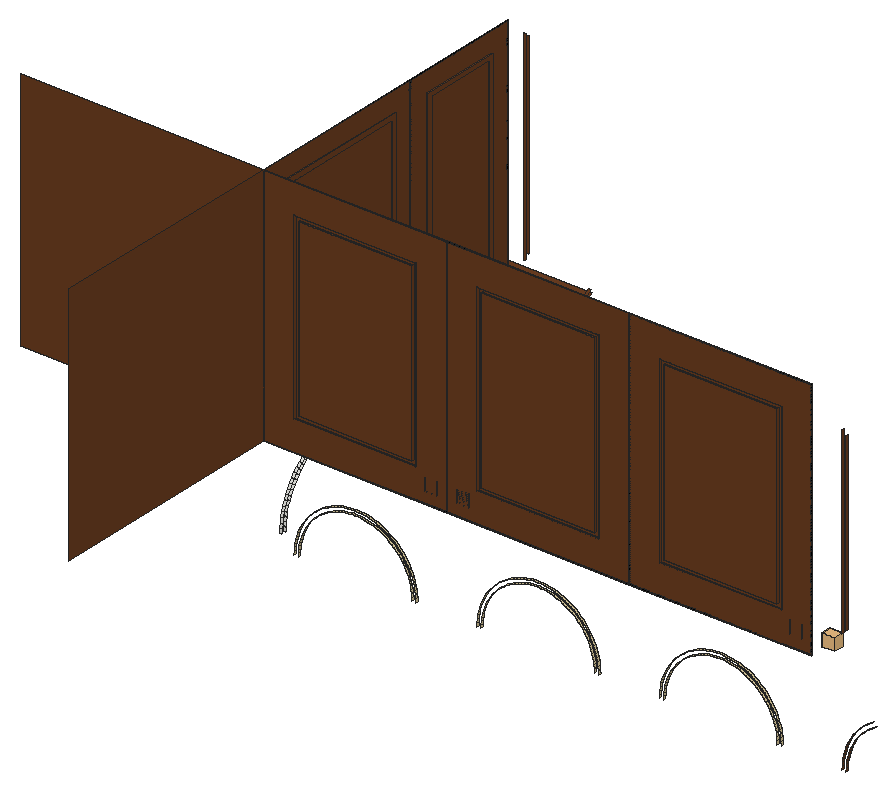
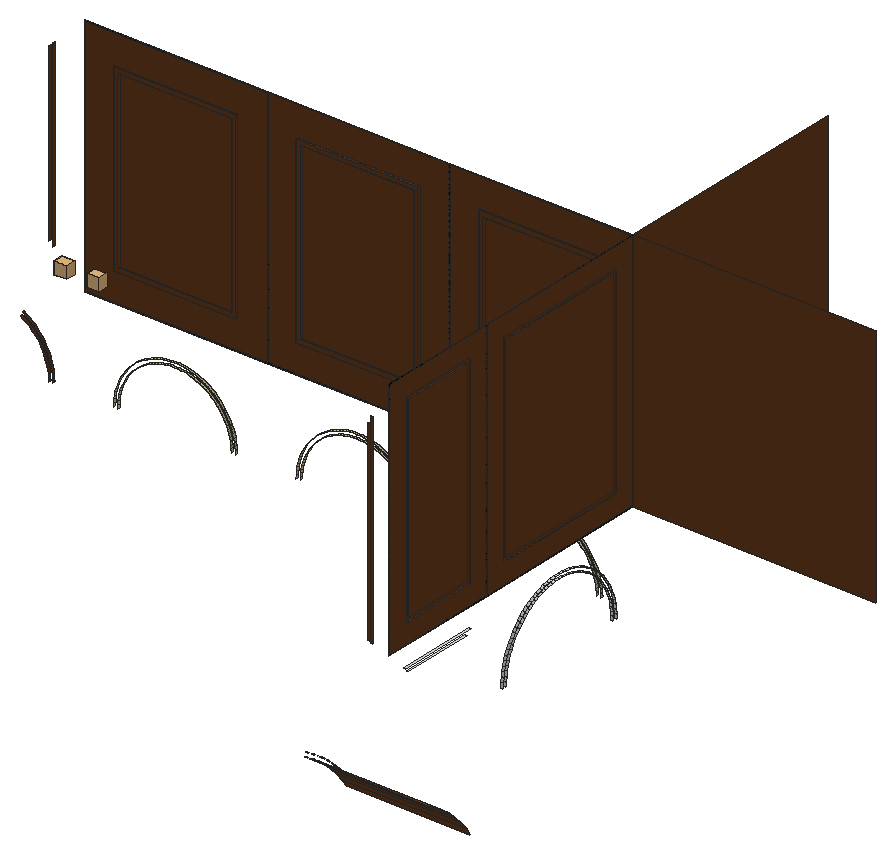
# SketchUp Ruby script. Lengths in inches.
U = 1.inch
M = Sketchup.active_model
def pt(a) = Geom::Point3d.new(a.map { |v| v * U })
def face(e, loops, mat)
  f = e.add_face(loops[0].map { |a| pt(a) })
  loops[1..].each { |l| e.add_face(l.map { |a| pt(a) }).erase! }
  f.material = f.back_material = mat if mat
  f
end
# faces: each face lists its corners as indices into pts; further lists are holes
def faces(e, pts, list, mat = nil) = list.each { |f| face(e, (f[0].is_a?(Array) ? f : [f]).map { |l| l.map { |i| pts[i] } }, mat) }
# xy, xz, yz: faces in a plane at the given z, y or x. An outline is a flat list of corners, or four numbers for a rectangle; further outlines are holes
def ring(l) = l.size == 4 ? [[l[0], l[1]], [l[2], l[1]], [l[2], l[3]], [l[0], l[3]]] : l.each_slice(2).to_a
def flat(e, list, mat, &to3) = list.each { |f| face(e, (f[0].is_a?(Array) ? f : [f]).map { |l| ring(l).map { |u, v| to3.(u, v) } }, mat) }
def xy(e, z, list, mat = nil) = flat(e, list, mat) { |x, y| [x, y, z] }
def xz(e, y, list, mat = nil) = flat(e, list, mat) { |x, z| [x, y, z] }
def yz(e, x, list, mat = nil) = flat(e, list, mat) { |y, z| [x, y, z] }
def lines(e, pts, list) = list.each { |a, b| e.add_line(pt(pts[a]), pt(pts[b])) }
# prism: a flat outline (further loops are holes) pulled along v
def prism(e, loops, v, mat = nil)
  f = face(e, loops, mat); d = Geom::Vector3d.new(v.map { |x| x * U })
  f.pushpull(f.normal.samedirection?(d) ? d.length : -d.length)
end
def box(e, o, s, mat = nil) = prism(e, [[o, [o[0] + s[0], o[1], o[2]], [o[0] + s[0], o[1] + s[1], o[2]], [o[0], o[1] + s[1], o[2]]]], [0, 0, s[2]], mat)
def at(x, y, z, deg = 0) = Geom::Transformation.translation(pt([x, y, z])) * Geom::Transformation.rotation(ORIGIN, Z_AXIS, deg.degrees)
def axes(o, x, y, z) = Geom::Transformation.new([*x, 0, *y, 0, *z, 0, *pt(o).to_a, 1])
def part(name) = M.definitions.add(name)
# library, detail: a bought-in or finely detailed component or shape, given as its bounding box
def library(name, o, s) = part(name).tap { |d| box(d.entities, o, s) }
def detail(e, o, s) = box(e.add_group.entities, o, s)
def put(e, d, t, mat = nil) = e.add_instance(d, t).tap { |i| i.material = mat if mat }
def group(e, t, mat = nil) = e.add_group.tap { |g| g.transformation = t; g.material = mat if mat }.entities
root = M.entities
M.materials.add("138_plaster painted wall texture-seamless").color = [214, 198, 153]
M.materials.add("[0137_Black]").color = [0, 0, 0]
M.materials.add("[Wood Veneer 01]").color = [104, 60, 32]
c1 = library("Group\#17",[0,0,0],[1.625,1.625,1.31])
xy(root,85.6,[[24,44.4,24.2,51.6]])
xy(root,86,[[24,44,24.2,52]])
xy(root,90,[[24,26,24.2,40],[24,44,24.2,52]],"[Wood Veneer 01]")
xy(root,90.4,[[24,26.4,24.2,39.6],[24,44.4,24.2,51.6]],"[Wood Veneer 01]")
xy(root,91,[[27,24,39,24.2],[45,24,57,24.2],[63,24,75,24.2]],"[Wood Veneer 01]")
xy(root,91.4,[[27.4,24,38.6,24.2],[45.4,24,56.6,24.2],[63.4,24,74.6,24.2]],"[Wood Veneer 01]")
xy(root,108.6,[[63.4,24,74.6,24.2]],"138_plaster painted wall texture-seamless")
xy(root,108.6,[[27.4,24,38.6,24.2],[45.4,24,56.6,24.2]],"[Wood Veneer 01]")
xy(root,109,[[27,24,39,24.2],[45,24,57,24.2],[63,24,75,24.2]],"[Wood Veneer 01]")
xy(root,109.6,[[24,26.4,24.2,39.6],[24,44.4,24.2,51.6]],"[Wood Veneer 01]")
xy(root,110,[[24,26,24.2,40],[24,44,24.2,52]],"[Wood Veneer 01]")
xz(root,24,[[[24,88,42,112],[24.1,88.1,41.9,111.9]],[[42,88,60,112],[42.1,88.1,59.9,111.9]],[[60,88,78,112],[60.1,88.1,77.9,111.9]]],"[0137_Black]")
xz(root,24,[[0,88,24,112],[[24.1,88.1,41.9,111.9],[27,91,39,109]],[[42.1,88.1,59.9,111.9],[45,91,57,109]],[[60.1,88.1,77.9,111.9],[63,91,75,109]],[27.4,91.4,38.6,108.6],
  [45.4,91.4,56.6,108.6],[63.4,91.4,74.6,108.6]],"[Wood Veneer 01]")
xz(root,24.2,[[[27,91,39,109],[27.4,91.4,38.6,108.6]],[[45,91,57,109],[45.4,91.4,56.6,108.6]],[[63,91,75,109],[63.4,91.4,74.6,108.6]]],"[Wood Veneer 01]")
xz(root,26,[[24,90,24.2,110]],"[Wood Veneer 01]")
xz(root,26.4,[[24,90.4,24.2,109.6]],"[Wood Veneer 01]")
xz(root,39.6,[[24,90.4,24.2,109.6]],"[Wood Veneer 01]")
xz(root,40,[[24,90,24.2,110]],"[Wood Veneer 01]")
xz(root,44,[[24,90,24.2,110]],"[Wood Veneer 01]")
xz(root,44.4,[[24,90.4,24.2,109.6]],"[Wood Veneer 01]")
xz(root,51.6,[[24,90.4,24.2,109.6]],"[Wood Veneer 01]")
xz(root,52,[[24,90,24.2,110]],"[Wood Veneer 01]")
xz(root,56,[[24,90,24.2,110]],"[Wood Veneer 01]")
xz(root,56.4,[[24,90.4,24.2,109.6]],"[Wood Veneer 01]")
yz(root,24,[[[24,88,42,112],[24.1,88.1,41.9,111.9]],[[42,88,54,112],[42.1,88.1,53.9,111.9]]],"[0137_Black]")
yz(root,24,[[0,88,24,112],[[24.1,88.1,41.9,111.9],[26,90,40,110]],[[42.1,88.1,53.9,111.9],[44,90,52,110]],[26.4,90.4,39.6,109.6],[44.4,90.4,51.6,109.6]],"[Wood Veneer 01]")
yz(root,24.2,[[[26,90,40,110],[26.4,90.4,39.6,109.6]],[[44,90,52,110],[44.4,90.4,51.6,109.6]]],"[Wood Veneer 01]")
yz(root,27,[[24,91,24.2,109]],"[Wood Veneer 01]")
yz(root,27.4,[[24,91.4,24.2,108.6]],"[Wood Veneer 01]")
yz(root,38.6,[[24,91.4,24.2,108.6]],"[Wood Veneer 01]")
yz(root,39,[[24,91,24.2,109]],"[Wood Veneer 01]")
yz(root,45,[[24,91,24.2,109]],"[Wood Veneer 01]")
yz(root,45.4,[[24,91.4,24.2,108.6]],"[Wood Veneer 01]")
yz(root,56.6,[[24,91.4,24.2,108.6]],"[Wood Veneer 01]")
yz(root,57,[[24,91,24.2,109]],"[Wood Veneer 01]")
yz(root,63,[[24,91,24.2,109]],"[Wood Veneer 01]")
yz(root,63.4,[[24,91.4,24.2,108.6]],"[Wood Veneer 01]")
yz(root,74.6,[[24,91.4,24.2,108.6]],"[Wood Veneer 01]")
yz(root,75,[[24,91,24.2,109]],"[Wood Veneer 01]")
yz(root,81,[[24,91,24.2,109]],"[Wood Veneer 01]")
yz(root,81.4,[[24,91.4,24.2,108.6]],"[Wood Veneer 01]")
p = [[12,59.625,79.5],[24.2,59.625,79.5],[24.2,59.03,78.67],[12,59.03,78.67],[24,59.31,79.74],[24,58.7,78.89],
  [24.2,58.7,78.89],[24.2,59.31,79.74],[27,24,79],[27.01,24,79.35],[27.01,24.2,79.35],[27,24.2,79],
  [27.41,24,79.33],[27.4,24,79],[27.4,24.2,79],[27.41,24.2,79.33],[38.6,24,79],[38.59,24,79.33],
  [38.59,24.2,79.33],[38.6,24.2,79],[38.99,24,79.35],[39,24,79],[39,24.2,79],[38.99,24.2,79.35],
  [45,24,79],[45.01,24,79.35],[45.01,24.2,79.35],[45,24.2,79],[45.41,24,79.33],[45.4,24,79],
  [45.4,24.2,79],[45.41,24.2,79.33],[56.6,24,79],[56.59,24,79.33],[56.59,24.2,79.33],[56.6,24.2,79],
  [56.99,24,79.35],[57,24,79],[57,24.2,79],[56.99,24.2,79.35],[63,24,79],[63.01,24,79.35],
  [63.01,24.2,79.35],[63,24.2,79],[63.41,24,79.33],[63.4,24,79],[63.4,24.2,79],[63.41,24.2,79.33],
  [74.6,24,79],[74.59,24,79.33],[74.59,24.2,79.33],[74.6,24.2,79],[74.99,24,79.35],[75,24,79],
  [75,24.2,79],[74.99,24.2,79.35],[81,24,79],[81.01,24,79.35],[81.01,24.2,79.35],[81,24.2,79],
  [81.41,24,79.33],[81.4,24,79],[81.4,24.2,79],[81.41,24.2,79.33],[24,26.01,79.46],[24,26,79],
  [24.2,26,79],[24.2,26.01,79.46],[24,26.4,79],[24,26.41,79.43],[24.2,26.41,79.43],[24.2,26.4,79],
  [24,39.59,79.43],[24,39.6,79],[24.2,39.6,79],[24.2,39.59,79.43],[24,40,79],[24,39.99,79.46],
  [24.2,39.99,79.46],[24.2,40,79],[27.04,24,79.7],[27.04,24.2,79.7],[27.4375,24,79.65],[27.4375,24.2,79.65],
  [38.5625,24,79.65],[38.5625,24.2,79.65],[38.96,24,79.7],[38.96,24.2,79.7],[45.04,24,79.7],[45.04,24.2,79.7],
  [45.4375,24,79.65],[45.4375,24.2,79.65],[56.5625,24,79.65],[56.5625,24.2,79.65],[56.96,24,79.7],[56.96,24.2,79.7],
  [63.04,24,79.7],[63.04,24.2,79.7],[63.4375,24,79.65],[63.4375,24.2,79.65],[74.5625,24,79.65],[74.5625,24.2,79.65],
  [74.96,24,79.7],[74.96,24.2,79.7],[81.04,24,79.7],[81.04,24.2,79.7],[81.4375,24,79.65],[81.4375,24.2,79.65],
  [24,26.46,79.86],[24.2,26.46,79.86],[24,39.54,79.86],[24.2,39.54,79.86],[24,26.06,79.91],[24.2,26.06,79.91],
  [24,39.94,79.91],[24.2,39.94,79.91],[12,60.27,80.29],[24.2,60.27,80.29],[27.09,24,80.04],[27.09,24.2,80.04],
  [27.49,24,79.97],[27.49,24.2,79.97],[38.51,24,79.97],[38.51,24.2,79.97],[38.91,24,80.04],[38.91,24.2,80.04],
  [45.09,24,80.04],[45.09,24.2,80.04],[45.49,24,79.97],[45.49,24.2,79.97],[56.51,24,79.97],[56.51,24.2,79.97],
  [56.91,24,80.04],[56.91,24.2,80.04],[63.09,24,80.04],[63.09,24.2,80.04],[63.49,24,79.97],[63.49,24.2,79.97],
  [74.51,24,79.97],[74.51,24.2,79.97],[74.91,24,80.04],[74.91,24.2,80.04],[81.09,24,80.04],[81.09,24.2,80.04],
  [81.49,24,79.97],[81.49,24.2,79.97],[24,59.97,80.55],[24.2,59.97,80.55],[24,26.13,80.37],[24.2,26.13,80.37],
  [24,26.53,80.29],[24.2,26.53,80.29],[24,39.47,80.29],[24.2,39.47,80.29],[24,39.87,80.37],[24.2,39.87,80.37],
  [27.16,24,80.38],[27.16,24.2,80.38],[27.55,24,80.29],[27.55,24.2,80.29],[38.45,24,80.29],[38.45,24.2,80.29],
  [38.84,24,80.38],[38.84,24.2,80.38],[45.16,24,80.38],[45.16,24.2,80.38],[45.55,24,80.29],[45.55,24.2,80.29],
  [56.45,24,80.29],[56.45,24.2,80.29],[56.84,24,80.38],[56.84,24.2,80.38],[63.16,24,80.38],[63.16,24.2,80.38],
  [63.55,24,80.29],[63.55,24.2,80.29],[74.45,24,80.29],[74.45,24.2,80.29],[74.84,24,80.38],[74.84,24.2,80.38],
  [81.16,24,80.38],[81.16,24.2,80.38],[81.55,24,80.29],[81.55,24.2,80.29],[27.64,24,80.61],[27.64,24.2,80.61],
  [38.36,24,80.61],[38.36,24.2,80.61],[45.64,24,80.61],[45.64,24.2,80.61],[56.36,24,80.61],[56.36,24.2,80.61],
  [63.64,24,80.61],[63.64,24.2,80.61],[74.36,24,80.61],[74.36,24.2,80.61],[81.64,24,80.61],[81.64,24.2,80.61],
  [24,26.625,80.71],[24.2,26.625,80.71],[24,39.375,80.71],[24.2,39.375,80.71],[12,60.97,81.03],[24.2,60.97,81.03],
  [27.25,24,80.72],[27.25,24.2,80.72],[38.75,24,80.72],[38.75,24.2,80.72],[45.25,24,80.72],[45.25,24.2,80.72],
  [56.75,24,80.72],[56.75,24.2,80.72],[63.25,24,80.72],[63.25,24.2,80.72],[74.75,24,80.72],[74.75,24.2,80.72],
  [81.25,24,80.72],[81.25,24.2,80.72],[24,26.24,80.8125],[24.2,26.24,80.8125],[24,39.76,80.8125],[24.2,39.76,80.8125],
  [24,60.6875,81.3125],[24.2,60.6875,81.3125],[27.74,24,80.92],[27.74,24.2,80.92],[38.26,24,80.92],[38.26,24.2,80.92],
  [45.74,24,80.92],[45.74,24.2,80.92],[56.26,24,80.92],[56.26,24.2,80.92],[63.74,24,80.92],[63.74,24.2,80.92],
  [74.26,24,80.92],[74.26,24.2,80.92],[81.74,24,80.92],[81.74,24.2,80.92],[27.36,24,81.05],[27.36,24.2,81.05],
  [38.64,24,81.05],[38.64,24.2,81.05],[45.36,24,81.05],[45.36,24.2,81.05],[56.64,24,81.05],[56.64,24.2,81.05],
  [63.36,24,81.05],[63.36,24.2,81.05],[74.64,24,81.05],[74.64,24.2,81.05],[81.36,24,81.05],[81.36,24.2,81.05],
  [24,26.75,81.12],[24.2,26.75,81.12],[24,39.25,81.12],[24.2,39.25,81.12],[24,26.37,81.25],[24.2,26.37,81.25],
  [24,39.63,81.25],[24.2,39.63,81.25],[27.86,24,81.22],[27.86,24.2,81.22],[38.14,24,81.22],[38.14,24.2,81.22],
  [45.86,24,81.22],[45.86,24.2,81.22],[56.14,24,81.22],[56.14,24.2,81.22],[63.86,24,81.22],[63.86,24.2,81.22],
  [74.14,24,81.22],[74.14,24.2,81.22],[81.86,24,81.22],[81.86,24.2,81.22],[12,61.71,81.73],[24.2,61.71,81.73],
  [27.49,24,81.375],[27.49,24.2,81.375],[38.51,24,81.375],[38.51,24.2,81.375],[45.49,24,81.375],[45.49,24.2,81.375],
  [56.51,24,81.375],[56.51,24.2,81.375],[63.49,24,81.375],[63.49,24.2,81.375],[74.51,24,81.375],[74.51,24.2,81.375],
  [81.49,24,81.375],[81.49,24.2,81.375],[24,26.9,81.53],[24.2,26.9,81.53],[24,39.1,81.53],[24.2,39.1,81.53],
  [28,24,81.51],[28,24.2,81.51],[38,24,81.51],[38,24.2,81.51],[46,24,81.51],[46,24.2,81.51],
  [56,24,81.51],[56,24.2,81.51],[64,24,81.51],[64,24.2,81.51],[74,24,81.51],[74,24.2,81.51],
  [82,24,81.51],[82,24.2,81.51],[24,26.53,81.68],[24.2,26.53,81.68],[24,39.47,81.68],[24.2,39.47,81.68],
  [24,61.45,82.03],[24.2,61.45,82.03],[27.64,24,81.69],[27.64,24.2,81.69],[38.36,24,81.69],[38.36,24.2,81.69],
  [45.64,24,81.69],[45.64,24.2,81.69],[56.36,24,81.69],[56.36,24.2,81.69],[63.64,24,81.69],[63.64,24.2,81.69],
  [74.36,24,81.69],[74.36,24.2,81.69],[81.64,24,81.69],[81.64,24.2,81.69],[28.15,24,81.8],[28.15,24.2,81.8],
  [37.85,24,81.8],[37.85,24.2,81.8],[46.15,24,81.8],[46.15,24.2,81.8],[55.85,24,81.8],[55.85,24.2,81.8],
  [64.15,24,81.8],[64.15,24.2,81.8],[73.85,24,81.8],[73.85,24.2,81.8],[82.15,24,81.8],[82.15,24.2,81.8],
  [24,27.08,81.92],[24.2,27.08,81.92],[24,38.92,81.92],[24.2,38.92,81.92],[27.8,24,82],[27.8,24.2,82],
  [38.2,24,82],[38.2,24.2,82],[45.8,24,82],[45.8,24.2,82],[56.2,24,82],[56.2,24.2,82],
  [63.8,24,82],[63.8,24.2,82],[74.2,24,82],[74.2,24.2,82],[81.8,24,82],[81.8,24.2,82],
  [24,26.72,82.1],[24.2,26.72,82.1],[24,39.28,82.1],[24.2,39.28,82.1],[12,62.5,82.375],[24.2,62.5,82.375],
  [28.32,24,82.08],[28.32,24.2,82.08],[37.68,24,82.08],[37.68,24.2,82.08],[46.32,24,82.08],[46.32,24.2,82.08],
  [55.68,24,82.08],[55.68,24.2,82.08],[64.32,24,82.08],[64.32,24.2,82.08],[73.68,24,82.08],[73.68,24.2,82.08],
  [82.32,24,82.08],[82.32,24.2,82.08],[24,27.28,82.3],[24.2,27.28,82.3],[24,38.72,82.3],[24.2,38.72,82.3],
  [27.99,24,82.3],[27.99,24.2,82.3],[38.01,24,82.3],[38.01,24.2,82.3],[45.99,24,82.3],[45.99,24.2,82.3],
  [56.01,24,82.3],[56.01,24.2,82.3],[63.99,24,82.3],[63.99,24.2,82.3],[74.01,24,82.3],[74.01,24.2,82.3],
  [81.99,24,82.3],[81.99,24.2,82.3],[24,62.26,82.69],[24.2,62.26,82.69],[28.51,24,82.34],[28.51,24.2,82.34],
  [37.49,24,82.34],[37.49,24.2,82.34],[46.51,24,82.34],[46.51,24.2,82.34],[55.49,24,82.34],[55.49,24.2,82.34],
  [64.51,24,82.34],[64.51,24.2,82.34],[73.49,24,82.34],[73.49,24.2,82.34],[82.51,24,82.34],[82.51,24.2,82.34],
  [24,26.9375,82.5],[24.2,26.9375,82.5],[24,39.0625,82.5],[24.2,39.0625,82.5],[28.1875,24,82.58],[28.1875,24.2,82.58],
  [28.71,24,82.6],[28.71,24.2,82.6],[37.29,24,82.6],[37.29,24.2,82.6],[37.8125,24,82.58],[37.8125,24.2,82.58],
  [46.1875,24,82.58],[46.1875,24.2,82.58],[46.71,24,82.6],[46.71,24.2,82.6],[55.29,24,82.6],[55.29,24.2,82.6],
  [55.8125,24,82.58],[55.8125,24.2,82.58],[64.1875,24,82.58],[64.1875,24.2,82.58],[64.71,24,82.6],[64.71,24.2,82.6],
  [73.29,24,82.6],[73.29,24.2,82.6],[73.8125,24,82.58],[73.8125,24.2,82.58],[82.1875,24,82.58],[82.1875,24.2,82.58],
  [82.71,24,82.6],[82.71,24.2,82.6],[24,27.51,82.67],[24.2,27.51,82.67],[24,38.49,82.67],[24.2,38.49,82.67],
  [12,63.33,82.97],[24.2,63.33,82.97],[24,27.18,82.89],[24.2,27.18,82.89],[24,38.82,82.89],[24.2,38.82,82.89],
  [28.4,24,82.86],[28.4,24.2,82.86],[28.93,24,82.84],[28.93,24.2,82.84],[37.07,24,82.84],[37.07,24.2,82.84],
  [37.6,24,82.86],[37.6,24.2,82.86],[46.4,24,82.86],[46.4,24.2,82.86],[46.93,24,82.84],[46.93,24.2,82.84],
  [55.07,24,82.84],[55.07,24.2,82.84],[55.6,24,82.86],[55.6,24.2,82.86],[64.4,24,82.86],[64.4,24.2,82.86],
  [64.93,24,82.84],[64.93,24.2,82.84],[73.07,24,82.84],[73.07,24.2,82.84],[73.6,24,82.86],[73.6,24.2,82.86],
  [82.4,24,82.86],[82.4,24.2,82.86],[82.93,24,82.84],[82.93,24.2,82.84],[24,27.76,83.02],[24.2,27.76,83.02],
  [24,38.24,83.02],[24.2,38.24,83.02],[24,63.11,83.3],[24.2,63.11,83.3],[29.16,24,83.07],[29.16,24.2,83.07],
  [36.84,24,83.07],[36.84,24.2,83.07],[47.16,24,83.07],[47.16,24.2,83.07],[54.84,24,83.07],[54.84,24.2,83.07],
  [65.16,24,83.07],[65.16,24.2,83.07],[72.84,24,83.07],[72.84,24.2,83.07],[83.16,24,83.07],[83.16,24.2,83.07],
  [28.64,24,83.12],[28.64,24.2,83.12],[37.36,24,83.12],[37.36,24.2,83.12],[46.64,24,83.12],[46.64,24.2,83.12],
  [55.36,24,83.12],[55.36,24.2,83.12],[64.64,24,83.12],[64.64,24.2,83.12],[73.36,24,83.12],[73.36,24.2,83.12],
  [82.64,24,83.12],[82.64,24.2,83.12],[24,27.45,83.26],[24.2,27.45,83.26],[24,38.55,83.26],[24.2,38.55,83.26],
  [24,28.04,83.35],[24.2,28.04,83.35],[24,37.96,83.35],[24.2,37.96,83.35],[12,64.2,83.51],[24.2,64.2,83.51],
  [28.88,24,83.36],[28.88,24.2,83.36],[29.4,24,83.29],[29.4,24.2,83.29],[36.6,24,83.29],[36.6,24.2,83.29],
  [37.12,24,83.36],[37.12,24.2,83.36],[46.88,24,83.36],[46.88,24.2,83.36],[47.4,24,83.29],[47.4,24.2,83.29],
  [54.6,24,83.29],[54.6,24.2,83.29],[55.12,24,83.36],[55.12,24.2,83.36],[64.88,24,83.36],[64.88,24.2,83.36],
  [65.4,24,83.29],[65.4,24.2,83.29],[72.6,24,83.29],[72.6,24.2,83.29],[73.12,24,83.36],[73.12,24.2,83.36],
  [82.88,24,83.36],[82.88,24.2,83.36],[83.4,24,83.29],[83.4,24.2,83.29],[29.66,24,83.49],[29.66,24.2,83.49],
  [36.34,24,83.49],[36.34,24.2,83.49],[47.66,24,83.49],[47.66,24.2,83.49],[54.34,24,83.49],[54.34,24.2,83.49],
  [65.66,24,83.49],[65.66,24.2,83.49],[72.34,24,83.49],[72.34,24.2,83.49],[83.66,24,83.49],[83.66,24.2,83.49],
  [24,27.74,83.62],[24.2,27.74,83.62],[24,38.26,83.62],[24.2,38.26,83.62],[24,64,83.86],[24.2,64,83.86],
  [29.14,24,83.6],[29.14,24.2,83.6],[36.86,24,83.6],[36.86,24.2,83.6],[47.14,24,83.6],[47.14,24.2,83.6],
  [54.86,24,83.6],[54.86,24.2,83.6],[65.14,24,83.6],[65.14,24.2,83.6],[72.86,24,83.6],[72.86,24.2,83.6],
  [83.14,24,83.6],[83.14,24.2,83.6],[24,28.33,83.67],[24.2,28.33,83.67],[24,37.67,83.67],[24.2,37.67,83.67],
  [29.92,24,83.68],[29.92,24.2,83.68],[36.08,24,83.68],[36.08,24.2,83.68],[47.92,24,83.68],[47.92,24.2,83.68],
  [54.08,24,83.68],[54.08,24.2,83.68],[65.92,24,83.68],[65.92,24.2,83.68],[72.08,24,83.68],[72.08,24.2,83.68],
  [83.92,24,83.68],[83.92,24.2,83.68],[29.42,24,83.8125],[29.42,24.2,83.8125],[36.58,24,83.8125],[36.58,24.2,83.8125],
  [47.42,24,83.8125],[47.42,24.2,83.8125],[54.58,24,83.8125],[54.58,24.2,83.8125],[65.42,24,83.8125],[65.42,24.2,83.8125],
  [72.58,24,83.8125],[72.58,24.2,83.8125],[83.42,24,83.8125],[83.42,24.2,83.8125],[24,28.05,83.95],[24.2,28.05,83.95],
  [24,37.95,83.95],[24.2,37.95,83.95],[30.2,24,83.85],[30.2,24.2,83.85],[35.8,24,83.85],[35.8,24.2,83.85],
  [48.2,24,83.85],[48.2,24.2,83.85],[53.8,24,83.85],[53.8,24.2,83.85],[66.2,24,83.85],[66.2,24.2,83.85],
  [71.8,24,83.85],[71.8,24.2,83.85],[84.2,24,83.85],[84.2,24.2,83.85],[24,28.65,83.96],[24.2,28.65,83.96],
  [24,37.35,83.96],[24.2,37.35,83.96],[29.7,24,84.01],[29.7,24.2,84.01],[30.49,24,84],[30.49,24.2,84],
  [35.51,24,84],[35.51,24.2,84],[36.3,24,84.01],[36.3,24.2,84.01],[47.7,24,84.01],[47.7,24.2,84.01],
  [48.49,24,84],[48.49,24.2,84],[53.51,24,84],[53.51,24.2,84],[54.3,24,84.01],[54.3,24.2,84.01],
  [65.7,24,84.01],[65.7,24.2,84.01],[66.49,24,84],[66.49,24.2,84],[71.51,24,84],[71.51,24.2,84],
  [72.3,24,84.01],[72.3,24.2,84.01],[83.7,24,84.01],[83.7,24.2,84.01],[24,28.38,84.26],[24.2,28.38,84.26],
  [24,37.62,84.26],[24.2,37.62,84.26],[30,24,84.2],[30,24.2,84.2],[30.78,24,84.14],[30.78,24.2,84.14],
  [35.22,24,84.14],[35.22,24.2,84.14],[36,24,84.2],[36,24.2,84.2],[48,24,84.2],[48,24.2,84.2],
  [48.78,24,84.14],[48.78,24.2,84.14],[53.22,24,84.14],[53.22,24.2,84.14],[54,24,84.2],[54,24.2,84.2],
  [66,24,84.2],[66,24.2,84.2],[66.78,24,84.14],[66.78,24.2,84.14],[71.22,24,84.14],[71.22,24.2,84.14],
  [72,24,84.2],[72,24.2,84.2],[84,24,84.2],[84,24.2,84.2],[24,28.98,84.24],[24.2,28.98,84.24],
  [24,37.02,84.24],[24.2,37.02,84.24],[31.08,24,84.26],[31.08,24.2,84.26],[34.92,24,84.26],[34.92,24.2,84.26],
  [49.08,24,84.26],[49.08,24.2,84.26],[52.92,24,84.26],[52.92,24.2,84.26],[67.08,24,84.26],[67.08,24.2,84.26],
  [70.92,24,84.26],[70.92,24.2,84.26],[30.31,24,84.36],[30.31,24.2,84.36],[35.69,24,84.36],[35.69,24.2,84.36],
  [48.31,24,84.36],[48.31,24.2,84.36],[53.69,24,84.36],[53.69,24.2,84.36],[66.31,24,84.36],[66.31,24.2,84.36],
  [71.69,24,84.36],[71.69,24.2,84.36],[24,29.33,84.49],[24.2,29.33,84.49],[24,36.67,84.49],[24.2,36.67,84.49],
  [31.39,24,84.36],[31.39,24.2,84.36],[34.61,24,84.36],[34.61,24.2,84.36],[49.39,24,84.36],[49.39,24.2,84.36],
  [52.61,24,84.36],[52.61,24.2,84.36],[67.39,24,84.36],[67.39,24.2,84.36],[70.61,24,84.36],[70.61,24.2,84.36],
  [24,28.74,84.55],[24.2,28.74,84.55],[24,37.26,84.55],[24.2,37.26,84.55],[30.625,24,84.51],[30.625,24.2,84.51],
  [31.71,24,84.45],[31.71,24.2,84.45],[32.03,24,84.51],[32.03,24.2,84.51],[34.29,24,84.45],[33.97,24,84.51],
  [33.97,24.2,84.51],[34.29,24.2,84.45],[35.375,24,84.51],[35.375,24.2,84.51],[48.625,24,84.51],[48.625,24.2,84.51],
  [49.71,24,84.45],[49.71,24.2,84.45],[50.03,24,84.51],[50.03,24.2,84.51],[52.29,24,84.45],[51.97,24,84.51],
  [51.97,24.2,84.51],[52.29,24.2,84.45],[53.375,24,84.51],[53.375,24.2,84.51],[66.625,24,84.51],[66.625,24.2,84.51],
  [67.71,24,84.45],[67.71,24.2,84.45],[68.03,24,84.51],[68.03,24.2,84.51],[70.29,24,84.45],[69.97,24,84.51],
  [69.97,24.2,84.51],[70.29,24.2,84.45],[71.375,24,84.51],[71.375,24.2,84.51],[30.95,24,84.64],[30.95,24.2,84.64],
  [32.35,24,84.5625],[32.35,24.2,84.5625],[33.65,24,84.5625],[33.65,24.2,84.5625],[35.05,24,84.64],[35.05,24.2,84.64],
  [48.95,24,84.64],[48.95,24.2,84.64],[50.35,24,84.5625],[50.35,24.2,84.5625],[51.65,24,84.5625],[51.65,24.2,84.5625],
  [53.05,24,84.64],[53.05,24.2,84.64],[66.95,24,84.64],[66.95,24.2,84.64],[68.35,24,84.5625],[68.35,24.2,84.5625],
  [69.65,24,84.5625],[69.65,24.2,84.5625],[71.05,24,84.64],[71.05,24.2,84.64],[24,29.7,84.72],[24.2,29.7,84.72],
  [24,36.3,84.72],[24.2,36.3,84.72],[31.28,24,84.75],[31.28,24.2,84.75],[32.67,24,84.59],[32.67,24.2,84.59],
  [33,24,84.6],[33,24.2,84.6],[33.33,24,84.59],[33.33,24.2,84.59],[34.72,24,84.75],[34.72,24.2,84.75],
  [49.28,24,84.75],[49.28,24.2,84.75],[50.67,24,84.59],[50.67,24.2,84.59],[51,24,84.6],[51,24.2,84.6],
  [51.33,24,84.59],[51.33,24.2,84.59],[52.72,24,84.75],[52.72,24.2,84.75],[67.28,24,84.75],[67.28,24.2,84.75],
  [68.67,24,84.59],[68.67,24.2,84.59],[69,24,84.6],[69,24.2,84.6],[69.33,24,84.59],[69.33,24.2,84.59],
  [70.72,24,84.75],[70.72,24.2,84.75],[24,29.11,84.82],[24.2,29.11,84.82],[24,36.89,84.82],[24.2,36.89,84.82],
  [31.62,24,84.84],[31.62,24.2,84.84],[34.38,24,84.84],[34.38,24.2,84.84],[49.62,24,84.84],[49.62,24.2,84.84],
  [52.38,24,84.84],[52.38,24.2,84.84],[67.62,24,84.84],[67.62,24.2,84.84],[70.38,24,84.84],[70.38,24.2,84.84],
  [24,30.08,84.92],[24.2,30.08,84.92],[24,35.92,84.92],[24.2,35.92,84.92],[31.96,24,84.91],[31.96,24.2,84.91],
  [34.04,24,84.91],[34.04,24.2,84.91],[49.96,24,84.91],[49.96,24.2,84.91],[52.04,24,84.91],[52.04,24.2,84.91],
  [67.96,24,84.91],[67.96,24.2,84.91],[70.04,24,84.91],[70.04,24.2,84.91],[24,29.5,85.0625],[24.2,29.5,85.0625],
  [24,36.5,85.0625],[24.2,36.5,85.0625],[32.3,24,84.96],[32.3,24.2,84.96],[33.7,24,84.96],[33.7,24.2,84.96],
  [50.3,24,84.96],[50.3,24.2,84.96],[51.7,24,84.96],[51.7,24.2,84.96],[68.3,24,84.96],[68.3,24.2,84.96],
  [69.7,24,84.96],[69.7,24.2,84.96],[24,30.47,85.1],[24.2,30.47,85.1],[24,35.53,85.1],[24.2,35.53,85.1],
  [32.65,24,84.99],[32.65,24.2,84.99],[33,24,85],[33,24.2,85],[33.35,24,84.99],[33.35,24.2,84.99],
  [50.65,24,84.99],[50.65,24.2,84.99],[51,24,85],[51,24.2,85],[51.35,24,84.99],[51.35,24.2,84.99],
  [68.65,24,84.99],[68.65,24.2,84.99],[69,24,85],[69,24.2,85],[69.35,24,84.99],[69.35,24.2,84.99],
  [24,29.9,85.28],[24.2,29.9,85.28],[24,30.88,85.25],[24.2,30.88,85.25],[24,35.12,85.25],[24.2,35.12,85.25],
  [24,36.1,85.28],[24.2,36.1,85.28],[24,31.29,85.375],[24.2,31.29,85.375],[24,34.71,85.375],[24.2,34.71,85.375],
  [24,30.32,85.47],[24.2,30.32,85.47],[24,35.68,85.47],[24.2,35.68,85.47],[24,31.71,85.47],[24.2,31.71,85.47],
  [24,34.29,85.47],[24.2,34.29,85.47],[24,30.75,85.63],[24.2,30.75,85.63],[24,32.14,85.54],[24.2,32.14,85.54],
  [24,32.57,85.59],[24.2,32.57,85.59],[24,33.43,85.59],[24,33.86,85.54],[24.2,33.86,85.54],[24.2,33.43,85.59],
  [24,35.25,85.63],[24.2,35.25,85.63],[24,31.1875,85.76],[24.2,31.1875,85.76],[24,33,85.6],[24.2,33,85.6],
  [24,34.8125,85.76],[24.2,34.8125,85.76],[24,31.63,85.87],[24.2,31.63,85.87],[24,34.37,85.87],[24.2,34.37,85.87],
  [24,32.09,85.94],[24.2,32.09,85.94],[24,32.54,85.99],[24.2,32.54,85.99],[24,33.91,85.94],[24,33.46,85.99],
  [24.2,33.46,85.99],[24.2,33.91,85.94],[24,33,86],[24.2,33,86]]
faces(root,p,[[0,1,2,3],[4,5,6,7],[56,57,58,59],[60,61,62,63],[57,104,105,58],[106,60,63,107],[116,117,1,0],[104,142,143,105],
  [144,106,107,145],[146,4,7,147],[142,180,181,143],[182,144,145,183],[196,182,183,197],[202,203,117,116],[180,216,217,181],[222,146,147,223],
  [236,196,197,237],[216,250,251,217],[272,236,237,273],[274,275,203,202],[250,288,289,251],[306,272,273,307],[312,222,223,313],[288,326,327,289],
  [340,306,307,341],[326,358,359,327],[364,365,275,274],[378,340,341,379],[358,396,397,359],[398,312,313,399],[412,378,379,413],[396,442,443,397],
  [444,412,413,445],[450,451,365,364],[442,480,481,443],[482,444,445,483],[488,398,399,489],[502,482,483,503],[480,516,517,481],[526,527,451,450],
  [516,552,553,517],[554,502,503,555],[568,554,555,569],[574,488,489,575],[552,588,589,553],[606,568,569,607],[588,620,621,589],[638,606,607,639],
  [620,668,669,621],[668,698,699,669]],"[Wood Veneer 01]")
faces(root,p,[[8,9,10,11],[12,13,14,15],[16,17,18,19],[20,21,22,23],[24,25,26,27],[28,29,30,31],[32,33,34,35],[36,37,38,39],
  [40,41,42,43],[44,45,46,47],[48,49,50,51],[52,53,54,55],[9,80,81,10],[82,12,15,83],[17,84,85,18],[86,20,23,87],
  [25,88,89,26],[90,28,31,91],[33,92,93,34],[94,36,39,95],[41,96,97,42],[98,44,47,99],[49,100,101,50],[102,52,55,103],
  [80,118,119,81],[120,82,83,121],[84,122,123,85],[124,86,87,125],[88,126,127,89],[128,90,91,129],[92,130,131,93],[132,94,95,133],
  [96,134,135,97],[136,98,99,137],[100,138,139,101],[140,102,103,141],[118,156,157,119],[158,120,121,159],[122,160,161,123],[162,124,125,163],
  [126,164,165,127],[166,128,129,167],[130,168,169,131],[170,132,133,171],[134,172,173,135],[174,136,137,175],[138,176,177,139],[178,140,141,179],
  [184,158,159,185],[160,186,187,161],[188,166,167,189],[168,190,191,169],[192,174,175,193],[176,194,195,177],[156,204,205,157],[206,162,163,207],
  [164,208,209,165],[210,170,171,211],[172,212,213,173],[214,178,179,215],[224,184,185,225],[186,226,227,187],[228,188,189,229],[190,230,231,191],
  [232,192,193,233],[194,234,235,195],[204,238,239,205],[240,206,207,241],[208,242,243,209],[244,210,211,245],[212,246,247,213],[248,214,215,249],
  [260,224,225,261],[226,262,263,227],[264,228,229,265],[230,266,267,231],[268,232,233,269],[234,270,271,235],[238,276,277,239],[278,240,241,279],
  [242,280,281,243],[282,244,245,283],[246,284,285,247],[286,248,249,287],[294,260,261,295],[262,296,297,263],[298,264,265,299],[266,300,301,267],
  [302,268,269,303],[270,304,305,271],[276,314,315,277],[316,278,279,317],[280,318,319,281],[320,282,283,321],[284,322,323,285],[324,286,287,325],
  [328,294,295,329],[296,330,331,297],[332,298,299,333],[300,334,335,301],[336,302,303,337],[304,338,339,305],[314,346,347,315],[348,316,317,349],
  [318,350,351,319],[352,320,321,353],[322,354,355,323],[356,324,325,357],[366,328,329,367],[330,368,369,331],[370,332,333,371],[334,372,373,335],
  [374,336,337,375],[338,376,377,339],[346,384,385,347],[386,348,349,387],[350,388,389,351],[390,352,353,391],[354,392,393,355],[394,356,357,395],
  [400,366,367,401],[368,402,403,369],[404,370,371,405],[372,406,407,373],[408,374,375,409],[376,410,411,377],[384,418,419,385],[420,400,401,421],
  [402,422,423,403],[424,386,387,425],[388,426,427,389],[428,404,405,429],[406,430,431,407],[432,390,391,433],[392,434,435,393],[436,408,409,437],
  [410,438,439,411],[440,394,395,441],[418,456,457,419],[458,420,421,459],[422,460,461,423],[462,424,425,463],[426,464,465,427],[466,428,429,467],
  [430,468,469,431],[470,432,433,471],[434,472,473,435],[474,436,437,475],[438,476,477,439],[478,440,441,479],[490,458,459,491],[460,492,493,461],
  [494,466,467,495],[468,496,497,469],[498,474,475,499],[476,500,501,477],[456,504,505,457],[506,462,463,507],[464,508,509,465],[510,470,471,511],
  [472,512,513,473],[514,478,479,515],[504,528,529,505],[530,490,491,531],[492,532,533,493],[534,506,507,535],[508,536,537,509],[538,494,495,539],
  [496,540,541,497],[542,510,511,543],[512,544,545,513],[546,498,499,547],[500,548,549,501],[550,514,515,551],[556,530,531,557],[532,558,559,533],
  [560,538,539,561],[540,562,563,541],[564,546,547,565],[548,566,567,549],[528,576,577,529],[578,534,535,579],[536,580,581,537],[582,542,543,583],
  [544,584,585,545],[586,550,551,587],[594,556,557,595],[558,596,597,559],[598,560,561,599],[562,600,601,563],[602,564,565,603],[566,604,605,567],
  [576,608,609,577],[610,578,579,611],[580,612,613,581],[614,582,583,615],[584,616,617,585],[618,586,587,619],[626,594,595,627],[596,628,629,597],
  [630,598,599,631],[600,632,633,601],[634,602,603,635],[604,636,637,605],[608,644,645,609],[646,626,627,647],[628,648,649,629],[650,610,611,651],
  [612,652,653,613],[654,630,631,655],[632,656,657,633],[658,614,615,659],[616,660,661,617],[662,634,635,663],[636,664,665,637],[666,618,619,667],
  [644,674,675,645],[676,646,647,677],[648,678,679,649],[680,650,651,681],[652,682,683,653],[684,654,655,685],[656,686,687,657],[688,658,659,689],
  [660,690,691,661],[692,662,663,693],[664,694,695,665],[696,666,667,697],[704,676,677,705],[678,706,707,679],[708,684,685,709],[686,710,711,687],
  [712,692,693,713],[694,714,715,695],[674,716,717,675],[718,680,681,719],[682,720,721,683],[722,688,689,723],[690,724,725,691],[726,696,697,727],
  [732,704,705,733],[706,734,735,707],[736,708,709,737],[710,738,739,711],[740,712,713,741],[714,742,743,715],[716,748,749,717],[750,732,733,751],
  [752,750,751,753],[754,755,756,757],[734,754,757,735],[758,718,719,759],[720,760,761,721],[762,736,737,763],[764,762,763,765],[766,767,768,769],
  [738,766,769,739],[770,722,723,771],[724,772,773,725],[774,740,741,775],[776,774,775,777],[778,779,780,781],[742,778,781,743],[782,726,727,783],
  [748,784,785,749],[786,752,753,787],[755,788,789,756],[790,758,759,791],[760,792,793,761],[794,764,765,795],[767,796,797,768],[798,770,771,799],
  [772,800,801,773],[802,776,777,803],[779,804,805,780],[806,782,783,807],[784,812,813,785],[814,786,787,815],[816,814,815,817],[818,816,817,819],
  [788,818,819,789],[820,790,791,821],[792,822,823,793],[824,794,795,825],[826,824,825,827],[828,826,827,829],[796,828,829,797],[830,798,799,831],
  [800,832,833,801],[834,802,803,835],[836,834,835,837],[838,836,837,839],[804,838,839,805],[840,806,807,841],[812,846,847,813],[848,820,821,849],
  [822,850,851,823],[852,830,831,853],[832,854,855,833],[856,840,841,857],[846,862,863,847],[864,848,849,865],[850,866,867,851],[868,852,853,869],
  [854,870,871,855],[872,856,857,873],[862,878,879,863],[880,864,865,881],[866,882,883,867],[884,868,869,885],[870,886,887,871],[888,872,873,889],
  [878,894,895,879],[894,896,897,895],[896,898,899,897],[898,880,881,899],[882,900,901,883],[900,902,903,901],[902,904,905,903],[904,884,885,905],
  [886,906,907,887],[906,908,909,907],[908,910,911,909],[910,888,889,911]],"138_plaster painted wall texture-seamless")
faces(root,p,[[64,65,66,67],[68,69,70,71],[72,73,74,75],[76,77,78,79],[69,108,109,70],[110,72,75,111],[112,64,67,113],[77,114,115,78],
  [148,112,113,149],[108,150,151,109],[152,110,111,153],[114,154,155,115],[150,198,199,151],[200,152,153,201],[218,148,149,219],[154,220,221,155],
  [198,252,253,199],[254,200,201,255],[256,218,219,257],[220,258,259,221],[252,290,291,253],[292,254,255,293],[308,256,257,309],[258,310,311,259],
  [290,342,343,291],[344,292,293,345],[360,308,309,361],[310,362,363,311],[342,380,381,343],[382,344,345,383],[414,360,361,415],[362,416,417,363],
  [380,446,447,381],[448,382,383,449],[452,414,415,453],[416,454,455,417],[446,484,485,447],[486,448,449,487],[518,452,453,519],[454,520,521,455],
  [484,522,523,485],[524,486,487,525],[570,518,519,571],[520,572,573,521],[522,590,591,523],[592,524,525,593],[622,570,571,623],[572,624,625,573],
  [590,640,641,591],[642,592,593,643],[670,622,623,671],[624,672,673,625],[640,700,701,641],[702,642,643,703],[700,728,729,701],[730,702,703,731],
  [744,670,671,745],[672,746,747,673],[728,808,809,729],[810,730,731,811],[842,744,745,843],[746,844,845,747],[808,858,859,809],[860,810,811,861],
  [874,842,843,875],[844,876,877,845],[858,890,891,859],[892,860,861,893],[912,874,875,913],[890,914,915,891],[916,892,893,917],[876,918,919,877],
  [914,920,921,915],[922,916,917,923],[924,912,913,925],[918,926,927,919],[920,928,929,921],[930,922,923,931],[932,924,925,933],[928,934,935,929],
  [934,936,937,935],[938,939,940,941],[939,930,931,940],[926,942,943,927],[944,932,933,945],[936,946,947,937],[946,938,941,947],[942,948,949,943],
  [950,944,945,951],[948,952,953,949],[954,950,951,955],[956,954,955,957],[958,959,960,961],[952,958,961,953],[962,956,957,963],[959,962,963,960]])
put(root,c1,axes([39.83,24,90.42],[0.75,0,0],[0,0,-0.75],[0,0.75,0]),"[Wood Veneer 01]")
put(root,c1,axes([43.02,24,90.42],[0.75,0,0],[0,0,-0.75],[0,0.75,0]),"[Wood Veneer 01]")
put(root,c1,axes([75.83,24,90.42],[0.75,0,0],[0,0,-0.75],[0,0.75,0]),"[Wood Veneer 01]")
put(root,c1,axes([79.02,24,90.42],[0.75,0,0],[0,0,-0.75],[0,0.75,0]),"[Wood Veneer 01]")
put(root,c1,axes([24,41.5625,89.82],[0,-0.74,0],[0,0,-0.74],[0.74,0,0]),"[Wood Veneer 01]")
put(root,c1,axes([24,43.6875,89.82],[0,-0.74,0],[0,0,-0.74],[0.74,0,0]),"[Wood Veneer 01]")
